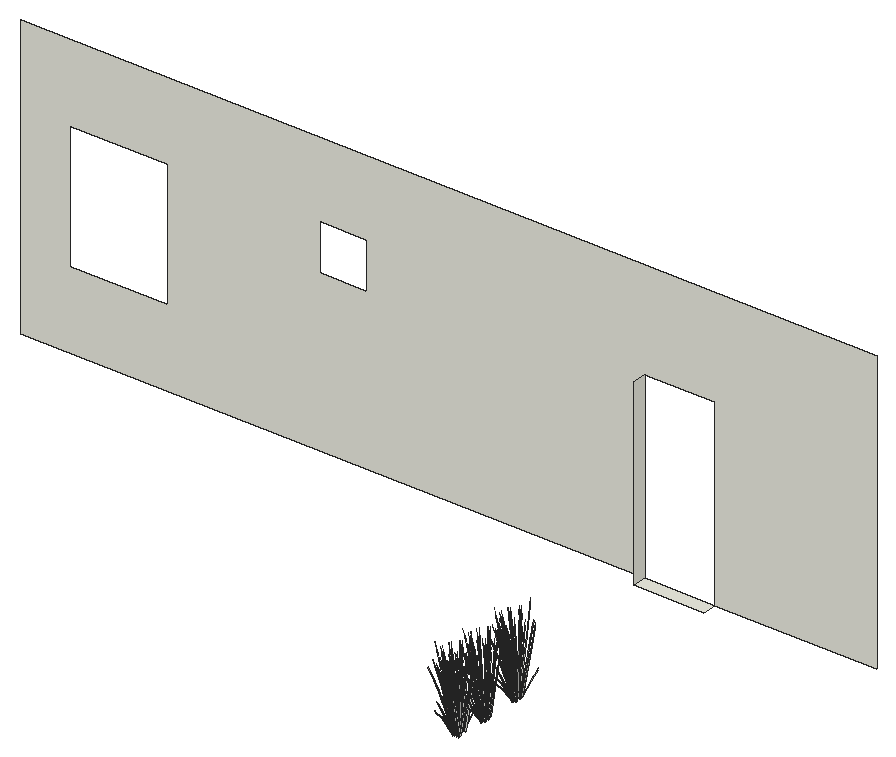
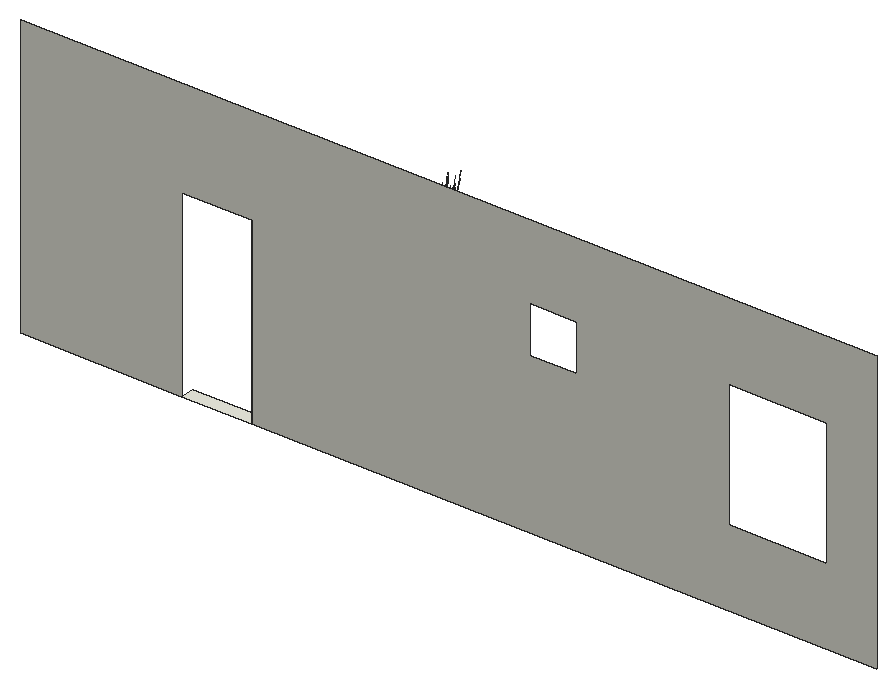
# SketchUp Ruby script. Lengths in inches.
U = 1.inch
M = Sketchup.active_model
def pt(a) = Geom::Point3d.new(a.map { |v| v * U })
def face(e, loops, mat)
  f = e.add_face(loops[0].map { |a| pt(a) })
  loops[1..].each { |l| e.add_face(l.map { |a| pt(a) }).erase! }
  f.material = f.back_material = mat if mat
  f
end
# faces: each face lists its corners as indices into pts; further lists are holes
def faces(e, pts, list, mat = nil) = list.each { |f| face(e, (f[0].is_a?(Array) ? f : [f]).map { |l| l.map { |i| pts[i] } }, mat) }
# xy, xz, yz: faces in a plane at the given z, y or x. An outline is a flat list of corners, or four numbers for a rectangle; further outlines are holes
def ring(l) = l.size == 4 ? [[l[0], l[1]], [l[2], l[1]], [l[2], l[3]], [l[0], l[3]]] : l.each_slice(2).to_a
def flat(e, list, mat, &to3) = list.each { |f| face(e, (f[0].is_a?(Array) ? f : [f]).map { |l| ring(l).map { |u, v| to3.(u, v) } }, mat) }
def xy(e, z, list, mat = nil) = flat(e, list, mat) { |x, y| [x, y, z] }
def xz(e, y, list, mat = nil) = flat(e, list, mat) { |x, z| [x, y, z] }
def yz(e, x, list, mat = nil) = flat(e, list, mat) { |y, z| [x, y, z] }
def lines(e, pts, list) = list.each { |a, b| e.add_line(pt(pts[a]), pt(pts[b])) }
# prism: a flat outline (further loops are holes) pulled along v
def prism(e, loops, v, mat = nil)
  f = face(e, loops, mat); d = Geom::Vector3d.new(v.map { |x| x * U })
  f.pushpull(f.normal.samedirection?(d) ? d.length : -d.length)
end
def box(e, o, s, mat = nil) = prism(e, [[o, [o[0] + s[0], o[1], o[2]], [o[0] + s[0], o[1] + s[1], o[2]], [o[0], o[1] + s[1], o[2]]]], [0, 0, s[2]], mat)
def at(x, y, z, deg = 0) = Geom::Transformation.translation(pt([x, y, z])) * Geom::Transformation.rotation(ORIGIN, Z_AXIS, deg.degrees)
def axes(o, x, y, z) = Geom::Transformation.new([*x, 0, *y, 0, *z, 0, *pt(o).to_a, 1])
def part(name) = M.definitions.add(name)
# library, detail: a bought-in or finely detailed component or shape, given as its bounding box
def library(name, o, s) = part(name).tap { |d| box(d.entities, o, s) }
def detail(e, o, s) = box(e.add_group.entities, o, s)
def put(e, d, t, mat = nil) = e.add_instance(d, t).tap { |i| i.material = mat if mat }
def group(e, t, mat = nil) = e.add_group.tap { |g| g.transformation = t; g.material = mat if mat }.entities
root = M.entities
M.materials.add("D01_Frost_White").color = [238, 238, 227]
M.materials.add("LightPink_Translucent").color = [144, 107, 117]
M.materials["LightPink_Translucent"].alpha = 0.75
c1 = part("blade")
p = [[2.15,0.21,22],[0,0.17,0],[0.09,0.45,0],[2.18,0.31,22],[2.29,0.31,22],[0.38,0.45,0],
  [2.48,0.24,33],[2.49,0.24,33],[2.48,0.22,33]]
faces(c1.entities,p,[[0,1,2,3],[4,5,2,3],[6,3,4,7],[8,0,3,6]])
c2 = part("seeds")
p = [[0.3,-0.1,1.38],[-0.01,-0.03,1.59],[-0.01,-0.03,0.03],[0.14,-0.07,-0.07],[0.29,-0.03,3],[0.15,0.01,3.11]]
faces(c2.entities,p,[[0,1,2,3],[1,0,4,5]],"LightPink_Translucent")
c3 = part("blade with seeds")
put(c3.entities,c1,at(0,0,0))
put(c3.entities,c2,axes([2.4,0.25,30.99],[1.5799,-0.05474,1.17369],[-0.12525,1.92788,0.29478],[-0.07173,-0.02425,1.56792]))
xy(root,150,[[277,361,307,367]],"D01_Frost_White")
xz(root,367,[[[10,150,10,270,376,270,376,150,307,150,307,228,277,228,277,150],[31,183,73,237],[138,218,158,238]]],"D01_Frost_White")
yz(root,277,[[361,150,367,228]],"D01_Frost_White")
put(root,c3,axes([294.12,243.97,150.27],[0.16998,-0.01068,1.44779],[-0.11276,0.46299,0.11706],[-0.24224,-0.02864,0.61892]))
put(root,c3,axes([294.1875,244.79,150.27],[0.14219,-0.09977,1.44779],[0.11971,0.461,0.11706],[-0.22323,0.10419,0.61892]))
put(root,c3,axes([294.875,274.63,150.27],[0.16998,-0.01068,1.44779],[-0.11276,0.46299,0.11706],[-0.24224,-0.02864,0.61892]))
put(root,c3,axes([293.75,244.625,150.98],[-0.06692,0.06124,1.47793],[0.00569,0.44742,-0.23373],[-0.15339,0.05818,0.11853]))
put(root,c3,axes([294.44,243.23,150.27],[0.15222,0.08126,1.44779],[-0.31502,0.34091,0.11706],[-0.19634,-0.15379,0.61892]))
put(root,c3,axes([294.95,275.44,150.27],[0.14219,-0.09977,1.44779],[0.11971,0.461,0.11706],[-0.22323,0.10419,0.61892]))
put(root,c3,axes([293.01,245.08,150.98],[0.0523,0.01265,1.49853],[0.16179,0.41674,-0.1416],[-0.10706,0.10938,0.26519]))
put(root,c3,axes([294.07,242.76,150.98],[0.03038,0.04707,1.49853],[-0.14646,0.42312,-0.1416],[-0.14833,0.00306,0.26519]))
put(root,c3,axes([295.59,257.02,150.27],[0.16998,-0.01068,1.44779],[-0.11276,0.46299,0.11706],[-0.24224,-0.02864,0.61892]))
put(root,c3,axes([294.41,242.48,150.98],[-0.08817,-0.00333,1.47793],[-0.28072,0.33293,-0.23373],[-0.14978,-0.06803,0.11853]))
put(root,c3,axes([294.05,244.32,151],[0.11578,-0.43006,0.40553],[0.38064,0.14706,0.33437],[-0.14969,0.02584,0.83914]))
put(root,c3,axes([294.18,244.2,151.25],[0.20619,0.42709,-0.10273],[-0.36595,0.20988,-0.57019],[-0.15422,0.05635,0.8664]))
put(root,c3,axes([294.65,243.3125,151.25],[-0.02194,0.47967,-0.10273],[-0.41546,-0.01311,-0.57019],[-0.16001,-0.03332,0.8664]))
put(root,c3,axes([294.51,275.28,150.98],[-0.06692,0.06124,1.47793],[0.00569,0.44742,-0.23373],[-0.15339,0.05818,0.11853]))
put(root,c3,axes([294.38,243.35,150.82],[-0.23317,-0.29531,-0.29918],[0.26625,-0.27955,0.38624],[-0.13527,-0.04253,0.73904]))
put(root,c3,axes([294.02,244.21,151],[-0.15051,-0.3216,0.05432],[0.27447,-0.15741,0.42765],[-0.12099,0.03106,0.65209]))
put(root,c3,axes([294.71,245.1,150.27],[0.10236,-0.14492,1.44779],[0.25844,0.39118,0.11706],[-0.17726,0.17814,0.61892]))
put(root,c3,axes([294.09,245.48,150.82],[-0.35672,0.06741,-0.29918],[-0.09419,-0.38534,0.38624],[-0.10222,0.1035,0.73904]))
put(root,c3,axes([294.73,275.03,150.82],[-0.34057,-0.13158,-0.29918],[0.09933,-0.38387,0.38624],[-0.13712,0.0352,0.73904]))
put(root,c3,axes([295.2,273.89,150.27],[0.15222,0.08126,1.44779],[-0.31502,0.34091,0.11706],[-0.19634,-0.15379,0.61892]))
put(root,c3,axes([295.66,257.84,150.27],[0.14219,-0.09977,1.44779],[0.11971,0.461,0.11706],[-0.22323,0.10419,0.61892]))
put(root,c3,axes([293.77,275.73,150.98],[0.0523,0.01265,1.49853],[0.16179,0.41674,-0.1416],[-0.10706,0.10938,0.26519]))
put(root,c3,axes([294.14,245.4,151],[-0.10163,-0.43409,0.40553],[0.39868,-0.07534,0.33437],[-0.1175,0.10209,0.83914]))
put(root,c3,axes([294.0625,245.3125,151],[-0.28133,-0.19836,0.05432],[0.16379,-0.28248,0.42765],[-0.0902,0.09132,0.65209]))
put(root,c3,axes([294.83,273.42,150.98],[0.03038,0.04707,1.49853],[-0.14646,0.42312,-0.1416],[-0.14833,0.00306,0.26519]))
put(root,c3,axes([294.63,245.46,150.27],[0.0763,-0.16212,1.44779],[0.3201,0.3355,0.11706],[-0.1444,0.2091,0.61892]))
put(root,c3,axes([295.17,273.14,150.98],[-0.08817,-0.00333,1.47793],[-0.28072,0.33293,-0.23373],[-0.14978,-0.06803,0.11853]))
put(root,c3,axes([294.33,244.33,151.27],[0.34057,0.13158,0.29918],[-0.09933,0.38387,-0.38624],[-0.13712,0.0352,0.73904]))
put(root,c3,axes([294.81,274.98,151],[0.11578,-0.43006,0.40553],[0.38064,0.14706,0.33437],[-0.14969,0.02584,0.83914]))
put(root,c3,axes([295.23,257.68,150.98],[-0.06692,0.06124,1.47793],[0.00569,0.44742,-0.23373],[-0.15339,0.05818,0.11853]))
put(root,c3,axes([294.94,274.85,151.25],[0.20619,0.42709,-0.10273],[-0.36595,0.20988,-0.57019],[-0.15422,0.05635,0.8664]))
put(root,c3,axes([295.41,273.97,151.25],[-0.02194,0.47967,-0.10273],[-0.41546,-0.01311,-0.57019],[-0.16001,-0.03332,0.8664]))
put(root,c3,axes([295.14,274,150.82],[-0.23317,-0.29531,-0.29918],[0.26625,-0.27955,0.38624],[-0.13527,-0.04253,0.73904]))
put(root,c3,axes([294.78,274.86,151],[-0.15051,-0.3216,0.05432],[0.27447,-0.15741,0.42765],[-0.12099,0.03106,0.65209]))
put(root,c3,axes([294.5,243.23,151],[0.02064,-0.35866,0.05432],[0.3116,0.00983,0.42765],[-0.11936,-0.03753,0.65209]))
put(root,c3,axes([293.76,246.3,150.98],[-0.01019,0.09334,1.47793],[0.28908,0.3247,-0.23373],[-0.07568,0.15355,0.11853]))
put(root,c3,axes([295.47,275.75,150.27],[0.10236,-0.14492,1.44779],[0.25844,0.39118,0.11706],[-0.17726,0.17814,0.61892]))
put(root,c3,axes([294.85,276.13,150.82],[-0.35672,0.06741,-0.29918],[-0.09419,-0.38534,0.38624],[-0.10222,0.1035,0.73904]))
put(root,c3,axes([295.46,242.61,151.59],[-0.2735,0.45217,-0.11506],[-0.39608,-0.2605,-0.63862],[-0.13768,-0.12775,0.97037]))
put(root,c3,axes([295.91,256.28,150.27],[0.15222,0.08126,1.44779],[-0.31502,0.34091,0.11706],[-0.19634,-0.15379,0.61892]))
put(root,c3,axes([294.71,243.5,151.27],[0.23317,0.29531,0.29918],[-0.26625,0.27955,-0.38624],[-0.13527,-0.04253,0.73904]))
put(root,c3,axes([294.48,258.13,150.98],[0.0523,0.01265,1.49853],[0.16179,0.41674,-0.1416],[-0.10706,0.10938,0.26519]))
put(root,c3,axes([294.9,276.05,151],[-0.10163,-0.43409,0.40553],[0.39868,-0.07534,0.33437],[-0.1175,0.10209,0.83914]))
put(root,c3,axes([294.2,245.22,151.25],[0.37908,0.26007,-0.10273],[-0.21839,0.37663,-0.57019],[-0.1071,0.13092,0.8664]))
put(root,c3,axes([294.82,275.97,151],[-0.28133,-0.19836,0.05432],[0.16379,-0.28248,0.42765],[-0.0902,0.09132,0.65209]))
put(root,c3,axes([295.54,255.8125,150.98],[0.03038,0.04707,1.49853],[-0.14646,0.42312,-0.1416],[-0.14833,0.00306,0.26519]))
put(root,c3,axes([295.39,276.11,150.27],[0.0763,-0.16212,1.44779],[0.3201,0.3355,0.11706],[-0.1444,0.2091,0.61892]))
put(root,c3,axes([295.88,255.53,150.98],[-0.08817,-0.00333,1.47793],[-0.28072,0.33293,-0.23373],[-0.14978,-0.06803,0.11853]))
put(root,c3,axes([295.52,257.37,151],[0.11578,-0.43006,0.40553],[0.38064,0.14706,0.33437],[-0.14969,0.02584,0.83914]))
put(root,c3,axes([294.38,245.25,151.27],[0.35672,-0.06741,0.29918],[0.09419,0.38534,-0.38624],[-0.10222,0.1035,0.73904]))
put(root,c3,axes([295.66,257.25,151.25],[0.20619,0.42709,-0.10273],[-0.36595,0.20988,-0.57019],[-0.15422,0.05635,0.8664]))
put(root,c3,axes([296.12,256.36,151.25],[-0.02194,0.47967,-0.10273],[-0.41546,-0.01311,-0.57019],[-0.16001,-0.03332,0.8664]))
put(root,c3,axes([295.49,257.26,151],[-0.15051,-0.3216,0.05432],[0.27447,-0.15741,0.42765],[-0.12099,0.03106,0.65209]))
put(root,c3,axes([296.18,258.15,150.27],[0.10236,-0.14492,1.44779],[0.25844,0.39118,0.11706],[-0.17726,0.17814,0.61892]))
put(root,c3,axes([295.26,273.89,151],[0.02064,-0.35866,0.05432],[0.3116,0.00983,0.42765],[-0.11936,-0.03753,0.65209]))
put(root,c3,axes([294.52,276.95,150.98],[-0.01019,0.09334,1.47793],[0.28908,0.3247,-0.23373],[-0.07568,0.15355,0.11853]))
put(root,c3,axes([296.22,273.27,151.59],[-0.2735,0.45217,-0.11506],[-0.39608,-0.2605,-0.63862],[-0.13768,-0.12775,0.97037]))
put(root,c3,axes([295.35,241.54,150.98],[-0.00765,0.05653,1.49853],[-0.37706,0.20517,-0.1416],[-0.11096,-0.10488,0.26519]))
put(root,c3,axes([294.72,246.27,151],[-0.29182,-0.32181,0.40553],[0.3099,-0.27755,0.33437],[-0.05383,0.15098,0.83914]))
put(root,c3,axes([295.61,258.44,151],[-0.10163,-0.43409,0.40553],[0.39868,-0.07534,0.33437],[-0.1175,0.10209,0.83914]))
put(root,c3,axes([295.22,242.68,150.82],[-0.06329,-0.37991,-0.29918],[0.36182,-0.10032,0.38624],[-0.09718,-0.10887,0.73904]))
put(root,c3,axes([294.61,246.24,151],[-0.33677,-0.02198,0.05432],[0.00923,-0.33185,0.42765],[-0.03524,0.12712,0.65209]))
put(root,c3,axes([294.96,275.87,151.25],[0.37908,0.26007,-0.10273],[-0.21839,0.37663,-0.57019],[-0.1071,0.13092,0.8664]))
put(root,c3,axes([295.53,258.36,151],[-0.28133,-0.19836,0.05432],[0.16379,-0.28248,0.42765],[-0.0902,0.09132,0.65209]))
put(root,c3,axes([294.72,246.37,150.82],[-0.27728,0.24833,-0.29918],[-0.26248,-0.28355,0.38624],[-0.03994,0.14407,0.73904]))
put(root,c3,axes([296.11,258.5,150.27],[0.0763,-0.16212,1.44779],[0.3201,0.3355,0.11706],[-0.1444,0.2091,0.61892]))
put(root,c3,axes([295.43,242.99,151.27],[0.06329,0.37991,0.29918],[-0.36182,0.10032,-0.38624],[-0.09718,-0.10887,0.73904]))
put(root,c3,axes([293.73,247.25,150.98],[0.04649,-0.02848,1.49853],[0.38427,0.18941,-0.1416],[-0.00903,0.15771,0.26519]))
put(root,c3,axes([295.8,257.38,151.27],[0.34057,0.13158,0.29918],[-0.09933,0.38387,-0.38624],[-0.13712,0.0352,0.73904]))
put(root,c3,axes([295.97,256.28,151],[0.02064,-0.35866,0.05432],[0.3116,0.00983,0.42765],[-0.11936,-0.03753,0.65209]))
put(root,c3,axes([295.24,259.35,150.98],[-0.01019,0.09334,1.47793],[0.28908,0.3247,-0.23373],[-0.07568,0.15355,0.11853]))
put(root,c3,axes([296.93,255.66,151.59],[-0.2735,0.45217,-0.11506],[-0.39608,-0.2605,-0.63862],[-0.13768,-0.12775,0.97037]))
put(root,c3,axes([296.11,272.19,150.98],[-0.00765,0.05653,1.49853],[-0.37706,0.20517,-0.1416],[-0.11096,-0.10488,0.26519]))
put(root,c3,axes([296.18,256.55,151.27],[0.23317,0.29531,0.29918],[-0.26625,0.27955,-0.38624],[-0.13527,-0.04253,0.73904]))
put(root,c3,axes([295.83,273.41,150.27],[0.09368,0.15143,1.44779],[-0.43286,0.12749,0.11706],[-0.09783,-0.23774,0.61892]))
put(root,c3,axes([295.375,242.64,151],[0.18625,-0.29962,0.05432],[0.26523,0.17444,0.42765],[-0.08575,-0.09606,0.65209]))
put(root,c3,axes([295.48,276.93,151],[-0.29182,-0.32181,0.40553],[0.3099,-0.27755,0.33437],[-0.05383,0.15098,0.83914]))
put(root,c3,axes([295.98,273.33,150.82],[-0.06329,-0.37991,-0.29918],[0.36182,-0.10032,0.38624],[-0.09718,-0.10887,0.73904]))
put(root,c3,axes([295.67,258.26,151.25],[0.37908,0.26007,-0.10273],[-0.21839,0.37663,-0.57019],[-0.1071,0.13092,0.8664]))
put(root,c3,axes([295.37,276.9,151],[-0.33677,-0.02198,0.05432],[0.00923,-0.33185,0.42765],[-0.03524,0.12712,0.65209]))
put(root,c3,axes([295.48,277.02,150.82],[-0.27728,0.24833,-0.29918],[-0.26248,-0.28355,0.38624],[-0.03994,0.14407,0.73904]))
put(root,c3,axes([294.49,277.91,150.98],[0.04649,-0.02848,1.49853],[0.38427,0.18941,-0.1416],[-0.00903,0.15771,0.26519]))
put(root,c3,axes([295.86,258.3,151.27],[0.35672,-0.06741,0.29918],[0.09419,0.38534,-0.38624],[-0.10222,0.1035,0.73904]))
put(root,c3,axes([294.87,246.02,151.27],[0.27728,-0.24833,0.29918],[0.26248,0.28355,-0.38624],[-0.03994,0.14407,0.73904]))
put(root,c3,axes([296.83,254.59,150.98],[-0.00765,0.05653,1.49853],[-0.37706,0.20517,-0.1416],[-0.11096,-0.10488,0.26519]))
put(root,c3,axes([294.6875,246.09,151.56],[0.45039,0.02337,-0.11403],[-0.01231,0.44247,-0.63292],[-0.03129,0.17041,0.9617]))
put(root,c3,axes([296.54,255.81,150.27],[0.09368,0.15143,1.44779],[-0.43286,0.12749,0.11706],[-0.09783,-0.23774,0.61892]))
put(root,c3,axes([296.42,242.77,151.25],[-0.40102,0.2196,-0.10273],[-0.19707,-0.38974,-0.57019],[-0.05291,-0.16424,0.8664]))
put(root,c3,axes([296.2,259.32,151],[-0.29182,-0.32181,0.40553],[0.3099,-0.27755,0.33437],[-0.05383,0.15098,0.83914]))
put(root,c3,axes([296.13,273.3,151],[0.18625,-0.29962,0.05432],[0.26523,0.17444,0.42765],[-0.08575,-0.09606,0.65209]))
put(root,c3,axes([295.33,245.8,150.27],[-0.01003,-0.18103,1.44779],[0.43473,0.12009,0.11706],[-0.02689,0.25798,0.61892]))
put(root,c3,axes([296.09,259.29,151],[-0.33677,-0.02198,0.05432],[0.00923,-0.33185,0.42765],[-0.03524,0.12712,0.65209]))
put(root,c3,axes([296.54,272.41,150.98],[-0.06268,-0.06613,1.47793],[-0.4183,0.04193,-0.23373],[-0.06676,-0.15817,0.11853]))
put(root,c3,axes([296.91,256.04,151.27],[0.06329,0.37991,0.29918],[-0.36182,0.10032,-0.38624],[-0.09718,-0.10887,0.73904]))
put(root,c3,axes([295.21,260.3,150.98],[0.04649,-0.02848,1.49853],[0.38427,0.18941,-0.1416],[-0.00903,0.15771,0.26519]))
put(root,c3,axes([296.3,242.93,151.27],[-0.12355,0.36271,0.29918],[-0.36044,-0.10579,-0.38624],[-0.03305,-0.14603,0.73904]))
put(root,c3,axes([295.45,276.74,151.56],[0.45039,0.02337,-0.11403],[-0.01231,0.44247,-0.63292],[-0.03129,0.17041,0.9617]))
put(root,c3,axes([295.53,246.76,151],[-0.30197,0.1603,0.05432],[-0.1478,-0.29231,0.42765],[0.02916,0.12885,0.65209]))
put(root,c3,axes([297.18,273.43,151.25],[-0.40102,0.2196,-0.10273],[-0.19707,-0.38974,-0.57019],[-0.05291,-0.16424,0.8664]))
put(root,c3,axes([296.85,255.69,151],[0.18625,-0.29962,0.05432],[0.26523,0.17444,0.42765],[-0.08575,-0.09606,0.65209]))
put(root,c3,axes([296.09,276.45,150.27],[-0.01003,-0.18103,1.44779],[0.43473,0.12009,0.11706],[-0.02689,0.25798,0.61892]))
put(root,c3,axes([297.25,254.8,150.98],[-0.06268,-0.06613,1.47793],[-0.4183,0.04193,-0.23373],[-0.06676,-0.15817,0.11853]))
put(root,c3,axes([296.26,242.55,150.82],[0.12355,-0.36271,-0.29918],[0.36044,0.10579,0.38624],[-0.03305,-0.14603,0.73904]))
put(root,c3,axes([295.68,246.81,150.82],[-0.12355,0.36271,-0.29918],[-0.36044,-0.10579,0.38624],[0.03305,0.14603,0.73904]))
put(root,c3,axes([296.34,259.07,151.27],[0.27728,-0.24833,0.29918],[0.26248,0.28355,-0.38624],[-0.03994,0.14407,0.73904]))
put(root,c3,axes([296.16,259.13,151.56],[0.45039,0.02337,-0.11403],[-0.01231,0.44247,-0.63292],[-0.03129,0.17041,0.9617]))
put(root,c3,axes([297.89,255.82,151.25],[-0.40102,0.2196,-0.10273],[-0.19707,-0.38974,-0.57019],[-0.05291,-0.16424,0.8664]))
put(root,c3,axes([296.41,242.6,151],[0.30197,-0.1603,0.05432],[0.1478,0.29231,0.42765],[-0.02916,-0.12885,0.65209]))
put(root,c3,axes([296.29,277.41,151],[-0.30197,0.1603,0.05432],[-0.1478,-0.29231,0.42765],[0.02916,0.12885,0.65209]))
put(root,c3,axes([295.43,247.45,150.98],[0.05195,0.07595,1.47793],[0.41921,0.02984,-0.23373],[0.04216,0.1675,0.11853]))
put(root,c3,axes([296.8,258.85,150.27],[-0.01003,-0.18103,1.44779],[0.43473,0.12009,0.11706],[-0.02689,0.25798,0.61892]))
put(root,c3,axes([296.3,242.63,151],[0.4038,0.12331,0.40553],[-0.13808,0.40538,0.33437],[-0.02427,-0.15942,0.83914]))
put(root,c3,axes([295.64,246.43,151.27],[0.12355,-0.36271,0.29918],[0.36044,0.10579,-0.38624],[0.03305,0.14603,0.73904]))
put(root,c3,axes([297.02,273.2,150.82],[0.12355,-0.36271,-0.29918],[0.36044,0.10579,0.38624],[-0.03305,-0.14603,0.73904]))
put(root,c3,axes([296.44,277.46,150.82],[-0.12355,0.36271,-0.29918],[-0.36044,-0.10579,0.38624],[0.03305,0.14603,0.73904]))
put(root,c3,axes([297.77,255.98,151.27],[-0.12355,0.36271,0.29918],[-0.36044,-0.10579,-0.38624],[-0.03305,-0.14603,0.73904]))
put(root,c3,axes([297,259.8,151],[-0.30197,0.1603,0.05432],[-0.1478,-0.29231,0.42765],[0.02916,0.12885,0.65209]))
put(root,c3,axes([295.52,246.58,151.25],[0.40102,-0.2196,-0.10273],[0.19707,0.38974,-0.57019],[0.05291,0.16424,0.8664]))
put(root,c3,axes([297.17,273.25,151],[0.30197,-0.1603,0.05432],[0.1478,0.29231,0.42765],[-0.02916,-0.12885,0.65209]))
put(root,c3,axes([296.1875,278.11,150.98],[0.05195,0.07595,1.47793],[0.41921,0.02984,-0.23373],[0.04216,0.1675,0.11853]))
put(root,c3,axes([297.57,242.23,150.98],[-0.04162,0.03603,1.49853],[-0.40776,-0.12155,-0.1416],[-0.01476,-0.15722,0.26519]))
put(root,c3,axes([297.25,243.27,151.25],[-0.45039,-0.02337,-0.10273],[0.01231,-0.44247,-0.57019],[0.03129,-0.17041,0.8664]))
put(root,c3,axes([297.06,273.28,151],[0.4038,0.12331,0.40553],[-0.13808,0.40538,0.33437],[-0.02427,-0.15942,0.83914]))
put(root,c3,axes([297.07,243.34,151.27],[-0.27728,0.24833,0.29918],[-0.26248,-0.28355,-0.38624],[0.03994,-0.14407,0.73904]))
put(root,c3,axes([296.64,246.63,151],[-0.4076,0.10824,0.40553],[-0.07074,-0.4246,0.33437],[0.09586,0.12514,0.83914]))
put(root,c3,axes([296.57,246.71,151],[-0.18625,0.29962,0.05432],[-0.26523,-0.17444,0.42765],[0.08575,0.09606,0.65209]))
